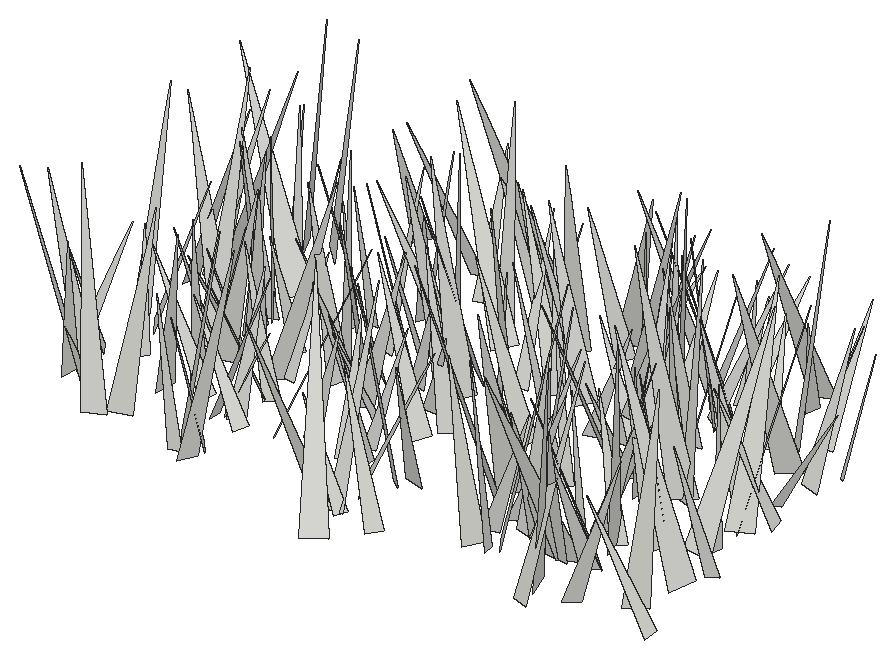
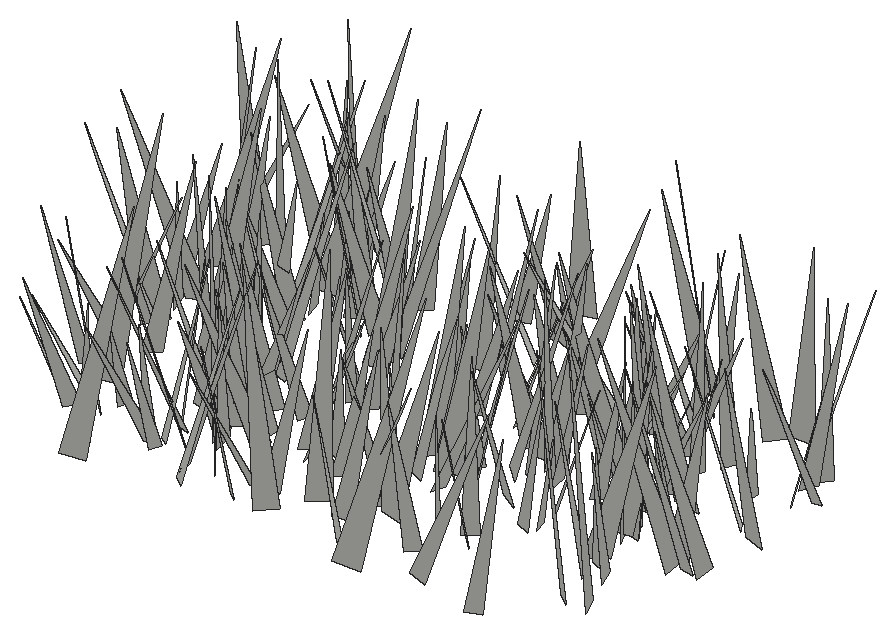
# SketchUp Ruby script. Lengths in inches.
U = 1.inch
M = Sketchup.active_model
def pt(a) = Geom::Point3d.new(a.map { |v| v * U })
def face(e, loops, mat)
  f = e.add_face(loops[0].map { |a| pt(a) })
  loops[1..].each { |l| e.add_face(l.map { |a| pt(a) }).erase! }
  f.material = f.back_material = mat if mat
  f
end
# faces: each face lists its corners as indices into pts; further lists are holes
def faces(e, pts, list, mat = nil) = list.each { |f| face(e, (f[0].is_a?(Array) ? f : [f]).map { |l| l.map { |i| pts[i] } }, mat) }
# xy, xz, yz: faces in a plane at the given z, y or x. An outline is a flat list of corners, or four numbers for a rectangle; further outlines are holes
def ring(l) = l.size == 4 ? [[l[0], l[1]], [l[2], l[1]], [l[2], l[3]], [l[0], l[3]]] : l.each_slice(2).to_a
def flat(e, list, mat, &to3) = list.each { |f| face(e, (f[0].is_a?(Array) ? f : [f]).map { |l| ring(l).map { |u, v| to3.(u, v) } }, mat) }
def xy(e, z, list, mat = nil) = flat(e, list, mat) { |x, y| [x, y, z] }
def xz(e, y, list, mat = nil) = flat(e, list, mat) { |x, z| [x, y, z] }
def yz(e, x, list, mat = nil) = flat(e, list, mat) { |y, z| [x, y, z] }
def lines(e, pts, list) = list.each { |a, b| e.add_line(pt(pts[a]), pt(pts[b])) }
# prism: a flat outline (further loops are holes) pulled along v
def prism(e, loops, v, mat = nil)
  f = face(e, loops, mat); d = Geom::Vector3d.new(v.map { |x| x * U })
  f.pushpull(f.normal.samedirection?(d) ? d.length : -d.length)
end
def box(e, o, s, mat = nil) = prism(e, [[o, [o[0] + s[0], o[1], o[2]], [o[0] + s[0], o[1] + s[1], o[2]], [o[0], o[1] + s[1], o[2]]]], [0, 0, s[2]], mat)
def at(x, y, z, deg = 0) = Geom::Transformation.translation(pt([x, y, z])) * Geom::Transformation.rotation(ORIGIN, Z_AXIS, deg.degrees)
def axes(o, x, y, z) = Geom::Transformation.new([*x, 0, *y, 0, *z, 0, *pt(o).to_a, 1])
def part(name) = M.definitions.add(name)
# library, detail: a bought-in or finely detailed component or shape, given as its bounding box
def library(name, o, s) = part(name).tap { |d| box(d.entities, o, s) }
def detail(e, o, s) = box(e.add_group.entities, o, s)
def put(e, d, t, mat = nil) = e.add_instance(d, t).tap { |i| i.material = mat if mat }
def group(e, t, mat = nil) = e.add_group.tap { |g| g.transformation = t; g.material = mat if mat }.entities
root = M.entities
c1 = part("fur_instance\#9")
p = [[0.8125,0,1.79],[0.67,-0.02,1.48],[0,-0.11,0],[0,0.11,0]]
faces(c1.entities,p,[[0,1,2,3]])
put(root,c1,axes([478.85,278.48,-21.66],[-3.36629,7.35026,0.38103],[7.33966,3.3212,0.77612],[-0.54849,-0.66835,8.0471]))
put(root,c1,axes([500.75,281.7,-21.66],[-4.62797,0.36048,0.06702],[0.36662,4.56134,0.78248],[0.00509,-0.78533,4.57556]))
put(root,c1,axes([492.17,282.21,-21.66],[7.07527,1.73735,2.55738],[2.12787,-7.36989,-0.88027],[-2.24293,-1.5114,7.23207]))
put(root,c1,axes([481.05,281.24,-21.66],[-3.33055,3.67395,0.98734],[3.8043,3.21801,0.85849],[0.0046,-1.30837,4.884]))
put(root,c1,axes([467.34,282.92,-21.66],[3.26712,2.26093,2.86418],[3.20778,-3.61207,-0.80776],[-1.73938,-2.41465,3.89016]))
put(root,c1,axes([478.22,281.67,-21.66],[-2.47066,2.78913,0.64805],[2.82871,2.24449,1.12431],[-0.44456,-1.21919,3.55237]))
put(root,c1,axes([466.3,281.52,-21.66],[-0.19493,4.51759,1.73565],[4.75586,-0.14282,0.90585],[-0.89608,-1.74071,4.43013]))
put(root,c1,axes([494.83,281.91,-21.66],[4.67154,-2.82363,0.84685],[-2.94301,-4.55853,1.0353],[-0.16964,1.32674,5.35951]))
put(root,c1,axes([467.43,281.26,-21.66],[6.54484,-1.1484,2.12677],[-1.53141,-6.71985,1.08414],[-1.86996,1.48383,6.55579]))
put(root,c1,axes([491.85,285.52,-21.66],[1.8393,-7.94223,0.20343],[-7.82957,-1.84746,-1.33722],[-1.34842,-0.10629,8.04201]))
put(root,c1,axes([465.96,282.625,-21.66],[6.04593,4.4435,2.18806],[4.86244,-5.98205,-1.28733],[-0.94282,-2.35709,7.39194]))
put(root,c1,axes([474.54,283.67,-21.66],[-1.00098,-5.50903,0.83943],[-5.47181,0.81017,-1.20786],[-1.05515,1.02481,5.46739]))
put(root,c1,axes([492.6,280.02,-21.66],[3.19327,6.60837,0.52108],[6.51338,-3.23542,1.11669],[-1.23207,0.02336,7.254]))
put(root,c1,axes([460.02,282.04,-21.66],[-1.69454,7.12423,1.83382],[7.32335,1.45532,1.11334],[-0.69716,-2.02889,7.23786]))
put(root,c1,axes([491.04,285.28,-21.66],[0.94954,-6.1364,0.24208],[-6.03443,-0.88683,1.18943],[1.14,0.41683,6.09444]))
put(root,c1,axes([486.33,283.63,-21.66],[-4.53938,3.59005,2.40826],[4.08452,4.7056,0.68422],[1.41595,-2.06469,5.74685]))
put(root,c1,axes([461.17,282.91,-21.66],[-3.27295,5.40819,2.7555],[5.57889,3.91368,-1.05481],[2.39109,-1.7286,6.23283]))
put(root,c1,axes([456.03,284.88,-21.66],[5.00192,-1.81934,1.03799],[-1.65,-5.07776,-0.94895],[-1.29032,-0.55947,5.23724]))
put(root,c1,axes([493.34,285.47,-21.66],[2.17041,-4.52553,0.56409],[-4.42394,-2.24099,-0.95709],[-1.10786,0.0828,4.92697]))
put(root,c1,axes([498.17,283.59,-21.66],[4.86014,-4.74094,2.82615],[-5.30574,-5.05065,0.65171],[-1.52079,2.46963,6.75816]))
put(root,c1,axes([457.46,284.31,-21.66],[-5.88104,-3.53705,0.94417],[-3.64814,5.81133,-0.9531],[0.30541,1.30636,6.79625]))
put(root,c1,axes([493.27,286.38,-21.66],[-4.06699,-5.2197,0.56162],[-5.13541,4.10303,0.94539],[1.09007,-0.14467,6.54919]))
put(root,c1,axes([487.39,283.66,-21.66],[-5.21816,-1.76906,1.50642],[-2.07355,5.2165,-1.05669],[1.04846,1.51216,5.4076]))
put(root,c1,axes([477.78,281.6875,-21.66],[1.53889,6.65129,0.3221],[6.53467,-1.57198,1.24039],[-1.28121,-0.02868,6.71336]))
put(root,c1,axes([488.67,286.82,-21.66],[4.29462,-4.11505,0.26594],[-3.98176,-4.23808,-1.27765],[-1.07236,-0.74374,5.80905]))
put(root,c1,axes([477.53,284.37,-21.66],[5.0651,3.0377,0.15182],[3.00547,-4.95362,-1.15532],[0.46672,-1.0677,5.79207]))
put(root,c1,axes([490.27,285.51,-21.66],[-1.57238,-4.56901,1.11948],[-4.65933,1.35009,-1.0341],[-0.64787,1.37945,4.72005]))
put(root,c1,axes([479.28,287,-21.66],[-0.0268,-5.65268,0.22398],[-5.53849,0.07185,1.15049],[1.15241,0.21383,5.53443]))
put(root,c1,axes([486.15,285.42,-21.66],[3.07396,-3.53335,0.83024],[-3.61315,-2.87553,1.13994],[0.34489,1.36741,4.5425]))
put(root,c1,axes([456.26,286.05,-21.66],[-6.02827,1.48886,1.73676],[1.72693,6.17226,0.7029],[1.50026,-1.12234,6.1695]))
put(root,c1,axes([461.34,286.85,-21.66],[5.97247,-1.71505,1.0533],[-1.60325,-6.04797,-0.7569],[-1.21673,-0.44932,6.16757]))
put(root,c1,axes([467.66,285.83,-21.66],[-3.1989,2.68909,0.37978],[2.66785,3.00183,1.21655],[-0.50792,-1.16886,3.99802]))
put(root,c1,axes([487.98,286.3,-21.66],[-0.07815,-6.05054,2.52953],[-6.4447,0.53908,1.09033],[1.2138,2.47266,5.952]))
put(root,c1,axes([487.625,284.45,-21.66],[6.38887,5.18246,1.59043],[5.07791,-6.58181,1.04866],[-1.89794,-0.16426,8.1594]))
put(root,c1,axes([497.56,287.66,-21.66],[4.54557,4.08977,3.87164],[5.12111,-5.0718,-0.65499],[-2.34307,-3.15097,6.07942]))
put(root,c1,axes([478.53,286.3125,-21.66],[2.96491,4.33641,3.25393],[4.46173,-4.05854,1.34327],[-3.07985,-1.70497,5.07846]))
put(root,c1,axes([484.5,288.24,-21.66],[-4.58981,-6.81856,1.14154],[-6.9132,4.53833,-0.68805],[0.05895,1.33156,8.19058]))
put(root,c1,axes([465.78,286.79,-21.66],[3.19259,1.80159,0.09548],[1.75198,-3.04965,-1.03811],[0.43061,-0.9494,3.51578]))
put(root,c1,axes([498.67,287.17,-21.66],[-7.81883,2.51294,1.68172],[2.76611,7.82758,1.16397],[1.22135,-1.64052,8.12983]))
put(root,c1,axes([471.63,287.34,-21.66],[1.56073,-4.1385,0.9971],[-4.17951,-1.28812,1.1957],[0.80812,1.33073,4.25833]))
put(root,c1,axes([465.54,286.11,-21.66],[4.89085,0.64493,0.58721],[0.56841,-4.89366,0.64042],[-0.66156,0.56328,4.89144]))
put(root,c1,axes([466.84,286.4375,-21.66],[-2.42701,4.03219,1.90827],[4.11447,2.86278,-0.81615],[1.72373,-1.15601,4.63496]))
put(root,c1,axes([484.32,289.6,-21.66],[5.05065,-5.78899,0.88016],[-5.66798,-5.12516,-1.18448],[-1.47008,-0.1285,7.59069]))
put(root,c1,axes([486.57,287.27,-21.66],[4.08139,-3.20586,0.61223],[-3.2526,-3.91407,1.18774],[0.27008,1.30866,5.05219]))
put(root,c1,axes([455.82,288.23,-21.66],[-3.08221,-2.2445,0.63722],[-2.14243,3.14072,0.69983],[0.92405,-0.20483,3.74807]))
put(root,c1,axes([463.95,287.48,-21.66],[-4.51711,1.79985,0.33219],[1.82954,4.41557,0.95372],[-0.05124,-1.00862,4.76803]))
put(root,c1,axes([464.62,285.65,-21.66],[4.77639,3.07128,1.21309],[2.81816,-4.90311,1.31748],[-1.72115,0.49496,5.52367]))
put(root,c1,axes([492.72,288.47,-21.66],[7.08469,1.17747,2.52447],[1.61288,-7.35894,-1.094],[-2.27113,-1.55299,7.09806]))
put(root,c1,axes([475.82,287.45,-21.66],[-4.15206,-1.52587,0.16301],[-1.50616,3.96212,-1.27574],[-0.29385,1.25209,4.2356]))
put(root,c1,axes([462.26,288.76,-21.66],[5.48977,-0.87036,1.92832],[-0.64898,-5.79667,-0.76876],[-2.01365,-0.50463,5.50492]))
put(root,c1,axes([454.75,287.21,-21.66],[1.35315,4.35582,0.79538],[4.34518,-1.14634,-1.11449],[0.85157,-1.07217,4.42291]))
put(root,c1,axes([474.34,286.75,-21.66],[-3.56654,2.39752,0.7344],[2.22273,3.6139,-1.00345],[1.16058,0.44646,4.17868]))
put(root,c1,axes([499.32,289.1,-21.66],[0.38107,-4.3176,1.24457],[-4.35966,-0.65774,-0.94692],[-1.08815,1.12319,4.22969]))
put(root,c1,axes([491.2,287.46,-21.66],[-4.4304,-0.23548,0.66281],[-0.42328,4.26855,-1.31284],[0.56178,1.35914,4.23796]))
put(root,c1,axes([469.55,286.65,-21.66],[5.6659,3.07924,0.02777],[3.03508,-5.59401,1.03936],[-0.52039,0.90013,6.36426]))
put(root,c1,axes([491.08,289.32,-21.66],[4.31446,-3.71791,0.40504],[-3.72385,-4.21342,0.9907],[0.3462,1.01276,5.60856]))
put(root,c1,axes([487.67,287.64,-21.66],[-4.49953,-3.59508,3.80394],[-4.60675,5.10137,-0.62788],[2.48443,2.94818,5.72505]))
put(root,c1,axes([494.8125,289.5625,-21.66],[4.62611,-3.05223,2.53258],[-2.97331,-5.24406,-0.88892],[-2.62479,0.5609,5.47054]))
put(root,c1,axes([492.79,288.73,-21.66],[1.4221,-3.78822,2.5832],[-4.25079,-2.10312,-0.74405],[-1.71882,2.06693,3.97736]))
put(root,c1,axes([466.5,289.45,-21.66],[-2.71564,-2.49022,0.0198],[-2.39499,2.6036,-1.03032],[-0.68234,0.77224,3.53756]))
put(root,c1,axes([473.71,290.93,-21.66],[-3.49973,-1.74713,0.54329],[-1.50598,3.41664,1.28623],[1.03907,-0.93268,3.69408]))
put(root,c1,axes([474.87,288.43,-21.66],[3.51726,-1.23078,1.44078],[-1.67757,-3.4351,1.16087],[-0.88116,1.62697,3.54095]))
put(root,c1,axes([467.04,289.42,-21.66],[1.69917,-3.99461,2.49122],[-4.30676,-2.38859,-0.89256],[-1.90128,1.84064,4.24822]))
put(root,c1,axes([484.5,290.53,-21.66],[0.91416,-4.94391,1.27953],[-4.9749,-1.15567,-0.91103],[-1.1532,1.06645,4.94449]))
put(root,c1,axes([458.07,288.97,-21.66],[-3.61922,1.27993,0.57976],[1.16278,3.62754,-0.74965],[0.78884,0.52519,3.76496]))
put(root,c1,axes([461.9,291.4,-21.66],[4.17452,-5.37379,1.20818],[-5.50555,-4.02647,1.11376],[0.16212,1.6352,6.71296]))
put(root,c1,axes([489.99,291.05,-21.66],[3.34433,-2.45993,0.06359],[-2.39384,-3.22746,1.0454],[0.56992,0.87868,4.01783]))
put(root,c1,axes([460.62,292.15,-21.66],[-3.9819,-2.09854,0.99873],[-1.89028,4.07705,1.03024],[1.35209,-0.4803,4.38155]))
put(root,c1,axes([470.4375,292.9,-21.66],[1.77342,-4.13167,0.71101],[-4.001,-1.89854,-1.053],[-1.2523,0.21471,4.37115]))
put(root,c1,axes([476.4,291.35,-21.66],[-4.85696,2.92878,0.85344],[3.03677,4.79447,0.82904],[0.29007,-1.15391,5.61075]))
put(root,c1,axes([462.3,292.6875,-21.66],[-0.70477,-3.63934,0.22038],[-3.52996,0.62491,-0.96896],[-0.91253,0.39339,3.57807]))
put(root,c1,axes([463.36,291.9375,-21.66],[-3.08913,-1.9262,0.20442],[-1.91689,2.98464,-0.84391],[-0.27849,0.82245,3.5413]))
put(root,c1,axes([465.73,291.59,-21.66],[6.31096,-2.97385,1.65761],[-3.28181,-6.24286,1.29466],[-0.9062,1.89806,6.85536]))
put(root,c1,axes([487.78,294.82,-21.66],[-3.38776,-6.42257,0.32475],[-6.36234,3.40084,0.88702],[0.93573,-0.12917,7.20691]))
put(root,c1,axes([456.41,292.04,-21.66],[4.70564,3.18962,0.73071],[3.27223,-4.59158,-1.02983],[-0.01227,-1.26267,5.59072]))
put(root,c1,axes([471.5,292.12,-21.66],[4.65487,-3.05281,1.35089],[-3.29302,-4.57961,0.99778],[-0.54826,1.58741,5.47649]))
put(root,c1,axes([466.07,291.91,-21.66],[-0.49271,4.25835,1.65602],[4.30491,0.99075,-1.26683],[1.53091,-1.41548,4.0953]))
put(root,c1,axes([490.07,294.01,-21.66],[3.94789,-1.4658,0.35037],[-1.34081,-3.86465,-1.06014],[-0.68816,-0.87925,4.0756]))
put(root,c1,axes([468.7,293.47,-21.66],[-5.74569,2.33772,2.68731],[2.89131,6.03979,0.92776],[2.08013,-1.9379,6.13328]))
put(root,c1,axes([497.58,291.7,-21.66],[-4.70779,-0.34884,1.44292],[-0.70643,4.74641,-1.15738],[1.30563,1.3103,4.57662]))
put(root,c1,axes([462.11,294.08,-21.66],[1.6892,-5.96403,1.00433],[-6.01842,-1.55459,0.89085],[0.59746,1.20222,6.13428]))
put(root,c1,axes([496.96,290.64,-21.66],[-0.59068,7.87895,1.19707],[7.83923,0.79048,-1.33468],[1.43434,-1.07565,7.78752]))
put(root,c1,axes([483.6,292.64,-21.66],[2.51167,3.62255,0.80621],[3.69421,-2.34748,-0.96099],[0.35452,-1.20325,4.30208]))
put(root,c1,axes([477.14,292.81,-21.66],[1.60632,-4.77246,2.92285],[-5.28453,-2.29441,-0.84211],[-1.84207,2.42054,4.96463]))
put(root,c1,axes([469.46,294.94,-21.66],[-2.94569,-5.43055,1.36405],[-5.282,3.20651,1.35919],[1.85796,0.50597,6.02666]))
put(root,c1,axes([474.76,294.08,-21.66],[1.46313,-3.34357,0.17988],[-3.25058,-1.37123,0.95187],[0.80348,0.54115,3.52337]))
put(root,c1,axes([488.31,293.77,-21.66],[4.57096,2.53062,0.74602],[2.63797,-4.36083,-1.37058],[0.04077,-1.55993,5.04174]))
put(root,c1,axes([482.78,294.48,-21.66],[3.65052,-1.24636,0.3015],[-1.17659,-3.61738,-0.70767],[-0.50984,-0.576,3.79195]))
put(root,c1,axes([486.3125,292.16,-21.66],[-4.58917,0.765,0.19448],[0.68534,4.43094,-1.25723],[0.3916,1.21042,4.47941]))
put(root,c1,axes([464.78,294.58,-21.66],[3.15907,-2.58161,1.45094],[-2.40771,-3.47422,-0.93937],[-1.72421,0.12146,3.97014]))
put(root,c1,axes([461.76,294.01,-21.66],[2.13967,5.72529,2.72362],[6.33838,-1.99885,-0.77766],[-0.14822,-2.82858,6.06237]))
put(root,c1,axes([484.8,293.13,-21.66],[-6.17227,-0.98801,0.5453],[-1.07692,6.06305,-1.2042],[0.3373,1.27815,6.13375]))
put(root,c1,axes([488.39,295.1,-21.66],[0.67909,-3.62862,0.46379],[-3.53581,-0.77205,-0.86319],[-0.93808,0.2832,3.58928]))
put(root,c1,axes([481.48,294.62,-21.66],[-5.50696,2.25656,1.40845],[2.52369,5.45565,1.12666],[0.84072,-1.59571,5.84374]))
put(root,c1,axes([492.36,295.125,-21.66],[2.49125,-7.31611,3.2771],[-7.62751,-3.2193,-1.38865],[-2.46697,2.5655,7.60286]))
put(root,c1,axes([470.43,295.32,-21.66],[-4.6315,-5.30606,1.24554],[-5.44783,4.55599,-0.84886],[0.16366,1.49838,6.99175]))
put(root,c1,axes([460.3,292.1,-21.66],[0.64716,8.27924,1.09317],[8.31403,-0.74193,0.69715],[-0.78591,-1.0312,8.27518]))
put(root,c1,axes([461.21,295.34,-21.66],[2.3019,2.88607,2.09295],[3.52279,-2.224,-0.8077],[-0.54756,-2.17555,3.60219]))
put(root,c1,axes([454.7,293.02,-21.66],[1.29784,6.7007,1.25957],[6.74597,-1.44798,0.75208],[-0.98888,-1.08363,6.78367]))
put(root,c1,axes([468.62,294.11,-21.66],[2.86323,5.98862,2.41998],[6.20716,-3.28322,0.78076],[-1.78634,-1.80966,6.59182]))
put(root,c1,axes([498.45,295.98,-21.66],[-4.68733,-0.90911,0.30449],[-0.85582,4.65242,0.7161],[0.43216,-0.64711,4.72067]))
put(root,c1,axes([472.43,295.88,-21.66],[0.98375,-3.96673,0.69714],[-3.91068,-0.76919,1.14174],[0.96305,0.9285,3.92417]))
put(root,c1,axes([467.69,294.625,-21.66],[-5.58164,-0.15602,0.84627],[-0.25003,5.60842,-0.61509],[0.82341,0.64537,5.54984]))
put(root,c1,axes([460.52,296.74,-21.66],[-2.8459,-6.01928,1.64103],[-5.98512,3.14324,1.14988],[1.76154,0.95508,6.5581]))
put(root,c1,axes([472.79,295.42,-21.66],[-4.95008,-4.07189,1.35786],[-4.2827,4.82407,-1.14641],[0.2873,1.75371,6.30629]))
put(root,c1,axes([474.5,296.41,-21.66],[-2.85824,2.70123,1.97363],[3.21945,2.92659,0.65696],[0.90938,-1.87078,3.87745]))
put(root,c1,axes([487.84,296.85,-21.66],[3.54062,0.10617,1.20258],[0.38468,-3.63127,-0.812],[-1.14433,-0.89222,3.44788]))
put(root,c1,axes([465.68,297.39,-21.66],[-3.61169,-1.5954,0.61372],[-1.41522,3.59542,1.01805],[0.9587,-0.70282,3.81487]))
put(root,c1,axes([497.0625,294.25,-21.66],[6.03648,4.13261,1.07509],[4.02235,-6.12795,0.97074],[-1.43354,0.20766,7.25088]))
put(root,c1,axes([495.21,297.11,-21.66],[4.87258,-2.82126,2.84071],[-2.53321,-5.63755,-1.25383],[-3.10033,0.17232,5.48903]))
put(root,c1,axes([475.28,296.43,-21.66],[-6.5147,3.53544,2.59254],[3.94464,6.75335,0.70282],[1.91322,-1.88542,7.3788]))
put(root,c1,axes([492.85,294.8,-21.66],[2.9733,6.47594,2.08154],[6.51847,-3.36189,1.14821],[-1.94427,-1.36785,7.03277]))
put(root,c1,axes([460.88,296.75,-21.66],[1.22573,-5.85041,2.29876],[-6.17569,-1.55733,-0.67049],[-1.1715,2.08841,5.93971]))
put(root,c1,axes([473.35,297.53,-21.66],[3.66547,-5.8791,2.24711],[-5.89364,-4.11869,-1.16204],[-2.20868,1.23351,6.83002]))
put(root,c1,axes([460.84,297.32,-21.66],[5.57047,2.74276,2.66238],[3.42235,-5.67452,-1.31471],[-1.7025,-2.43273,6.06831]))
put(root,c1,axes([497.28,294.17,-21.66],[-5.06165,5.7028,1.49455],[5.55918,5.27278,-1.292],[1.96243,-0.22764,7.51486]))
put(root,c1,axes([474.52,298.93,-21.66],[-3.9391,-6.11846,0.96009],[-6.01065,4.05101,1.1555],[1.49311,0.1661,7.18449]))
put(root,c1,axes([457.06,296.97,-21.66],[1.7878,3.1828,1.34143],[3.44443,-1.53093,-0.95817],[0.2561,-1.62848,3.52255]))
put(root,c1,axes([489.68,297.91,-21.66],[-1.49561,-5.63035,1.67127],[-5.71638,1.79132,0.91926],[1.34798,1.34949,5.75262]))
put(root,c1,axes([470.625,298.5625,-21.66],[-3.85431,-2.63258,1.04926],[-2.43046,3.98156,1.06172],[1.4575,-0.32233,4.54521]))
put(root,c1,axes([485.56,297.93,-21.66],[2.4486,-4.30122,0.69777],[-4.269,-2.2075,1.37318],[0.8735,1.26866,4.75506]))
put(root,c1,axes([457.02,297.09,-21.66],[-2.59565,5.50063,1.7013],[5.74289,2.3395,1.19781],[-0.41302,-2.03926,5.96319]))
put(root,c1,axes([487.13,297.68,-21.66],[-3.1283,2.85302,0.75954],[2.94685,2.94951,1.058],[-0.18092,-1.28978,4.09959]))
put(root,c1,axes([483.6875,297.57,-21.66],[3.11489,-2.67244,0.85057],[-2.80172,-2.90834,1.1224],[0.12545,1.40269,3.94774]))
put(root,c1,axes([488.51,296.26,-21.66],[-5.11212,3.73872,1.49873],[3.53116,5.32488,-1.23875],[1.93782,0.15985,6.21106]))
put(root,c1,axes([454.67,297.48,-21.66],[6.22243,-0.20354,0.93497],[-0.30289,-6.25415,0.65425],[-0.90767,0.69164,6.19128]))
put(root,c1,axes([476.15,299.46,-21.66],[-2.86307,-5.78602,1.82095],[-5.78172,3.21211,1.11581],[1.83453,1.09334,6.35847]))
put(root,c1,axes([472.6,299.3,-21.66],[-6.27523,-0.24227,0.55286],[-0.1392,6.19931,1.13667],[0.58735,-1.11924,6.17618]))
put(root,c1,axes([497.02,297.79,-21.66],[3.6219,-1.04912,0.12415],[-1.02885,-3.40219,1.26523],[0.23987,1.24847,3.55218]))
put(root,c1,axes([495.21,301.28,-21.66],[3.52334,-7.25518,1.10129],[-7.15699,-3.66725,-1.26216],[-1.62106,0.42196,7.96608]))
put(root,c1,axes([476.77,297.96,-21.66],[1.67627,3.15128,1.04901],[3.10636,-1.90337,0.75402],[-1.17538,-0.53615,3.48882]))
put(root,c1,axes([455.6,297.99,-21.66],[2.77668,6.00015,1.42785],[6.14966,-2.57364,-1.14395],[0.47149,-1.76779,6.51177]))
put(root,c1,axes([456.45,298,-21.66],[7.58645,0.4489,1.20084],[0.2907,-7.62155,1.01257],[-1.24861,0.95304,7.53196]))
put(root,c1,axes([465.38,299.07,-21.66],[-3.65849,-0.26653,0.63033],[-0.40108,3.61269,-0.80033],[0.55452,0.85461,3.57982]))
put(root,c1,axes([468.625,297.9,-21.66],[1.97963,5.14738,0.61551],[5.06452,-2.06097,0.94673],[-1.10678,-0.22402,5.43306]))
put(root,c1,axes([466.03,299.85,-21.66],[-1.43157,-3.77915,1.63266],[-4.11341,1.2436,-0.72817],[-0.16553,1.78,3.97506]))
put(root,c1,axes([489.01,300.27,-21.66],[-0.52973,-5.32119,2.08202],[-5.65742,0.19488,-0.94137],[-0.8022,2.1395,5.26399]))
put(root,c1,axes([489.66,298.7,-21.66],[4.69636,2.95892,0.9191],[2.85112,-4.78039,0.82137],[-1.21287,0.21986,5.48965]))
put(root,c1,axes([481.15,300.29,-21.66],[-4.7653,3.97573,1.88545],[4.327,4.73874,0.94381],[0.79899,-1.95123,6.13381]))
put(root,c1,axes([460.6,299.96,-21.66],[-6.11884,4.72961,1.11538],[4.85918,5.97068,1.339],[0.0418,-1.7422,7.61686]))
put(root,c1,axes([467.91,302.25,-21.66],[4.2644,-2.86076,0.08373],[-2.8192,-4.22473,-0.76148],[-0.49304,-0.58632,5.07831]))
put(root,c1,axes([486.15,300.71,-21.66],[-1.6675,3.7386,1.84502],[3.94069,2.06209,-0.61692],[1.36097,-1.39013,4.04687]))
put(root,c1,axes([480.8125,300.8,-21.66],[-5.83458,-0.97839,0.23219],[-1.00024,5.78729,-0.74851],[0.10327,0.77686,5.8685]))
put(root,c1,axes([459.8,301.95,-21.66],[5.00049,1.26706,0.71261],[1.41038,-4.84715,-1.27832],[-0.35226,-1.4205,4.99762]))
put(root,c1,axes([483.9,300.7,-21.66],[7.6269,-0.50277,1.8471],[-0.68475,-7.80192,0.70374],[-1.78765,0.84341,7.61099]))
put(root,c1,axes([497.23,300.5,-21.66],[0.7475,5.23214,1.319],[5.34274,-0.53135,-0.92008],[0.75507,-1.41992,5.20456]))
put(root,c1,axes([486.23,299.77,-21.66],[-5.56085,2.56326,1.5764],[2.25423,5.74256,-1.38556],[1.99343,0.65656,5.96435]))
put(root,c1,axes([479.32,300.09,-21.66],[-0.14147,5.00237,0.6936],[4.87308,-0.04695,1.33257],[-1.32587,-0.70632,4.82369]))
put(root,c1,axes([477.17,299.35,-21.66],[0.66443,5.27954,0.01832],[5.19176,-0.65673,0.9642],[-0.95891,0.10252,5.2331]))
put(root,c1,axes([486.18,302.52,-21.66],[7.03768,2.72348,2.80411],[3.28727,-7.24831,-1.21043],[-2.11523,-2.20318,7.44856]))
put(root,c1,axes([477.89,301.53,-21.66],[-4.17135,3.80631,1.04328],[3.93898,4.10999,0.75433],[0.24669,-1.26356,5.59635]))
put(root,c1,axes([459.77,300.73,-21.66],[0.78619,5.10987,0.99795],[4.99569,-1.02461,1.31074],[-1.46621,-0.75112,5.00108]))
put(root,c1,axes([484.43,301.3125,-21.66],[-4.83197,-1.5354,1.95575],[-2.0901,4.8234,-1.3772],[1.34681,1.9768,4.87942]))
put(root,c1,axes([458.76,301.4,-21.66],[-4.7564,-0.43454,1.78324],[-0.95829,4.81251,-1.3833],[1.56539,1.62573,4.5715]))
put(root,c1,axes([488.3,304.64,-21.66],[-3.60567,-4.25836,0.82426],[-4.10665,3.69659,1.13335],[1.39586,-0.12438,5.46351]))
put(root,c1,axes([488.5625,302.73,-21.66],[3.89411,3.28531,3.07479],[3.51498,-4.75969,0.63397],[-2.80935,-1.40135,5.05524]))
put(root,c1,axes([477.09,304.58,-21.66],[5.45655,-4.97036,1.37233],[-4.9464,-5.60993,-0.6508],[-1.45634,0.43117,7.35221]))
put(root,c1,axes([483.26,301.95,-21.66],[6.3266,0.04535,0.7535],[-0.10627,-6.24313,1.26797],[-0.74735,1.27161,6.1984]))
put(root,c1,axes([473.5,302.51,-21.66],[-6.02819,4.2729,0.70004],[4.32885,5.97346,0.81585],[0.09372,-1.07093,7.34378]))
put(root,c1,axes([486.41,301.68,-21.66],[-2.91269,3.59929,0.76549],[3.33369,2.99435,-1.39463],[1.55801,0.3218,4.41516]))
put(root,c1,axes([485.46,302.79,-21.66],[-5.53054,0.45224,1.5037],[0.10523,5.59989,-1.29715],[1.5667,1.22031,5.39525]))
put(root,c1,axes([498.01,302.51,-21.66],[2.52886,2.74781,0.4271],[2.47453,-2.48701,1.34889],[-1.2687,0.62635,3.48225]))
put(root,c1,axes([488.21,302.99,-21.66],[2.55836,5.15566,0.46861],[5.11042,-2.43162,-1.14739],[0.82709,-0.92305,5.63999]))
put(root,c1,axes([492.64,302.73,-21.66],[-3.06168,2.49465,0.02952],[2.42804,2.99025,-0.87237],[0.57338,0.65813,3.85176]))
put(root,c1,axes([474.75,305.39,-21.66],[1.57492,-4.967,1.49516],[-5.0252,-1.8484,-0.84719],[-1.28605,1.13987,5.14138]))
put(root,c1,axes([457.36,304.64,-21.66],[6.90611,3.10223,2.59996],[3.46907,-7.18559,-0.64093],[-2.08547,-1.6797,7.5437]))
put(root,c1,axes([467.46,303.14,-21.66],[2.96652,3.66752,1.13191],[3.55325,-3.16507,0.94281],[-1.45132,-0.25254,4.62191]))
put(root,c1,axes([459.15,304.81,-21.66],[-4.14785,-5.45032,3.6874],[-5.74845,5.12259,1.10541],[3.20285,2.13555,6.75935]))
put(root,c1,axes([472.67,303.52,-21.66],[0.75585,6.87514,1.87347],[7.05211,-0.99202,0.79528],[-1.02238,-1.75986,6.87069]))
put(root,c1,axes([479.79,305.66,-21.66],[3.58153,-3.37168,2.12142],[-3.21603,-4.13077,-1.13573],[-2.3507,0.51427,4.78599]))
put(root,c1,axes([485.39,306.39,-21.66],[-6.52757,-2.25287,1.08541],[-2.07972,6.57544,1.14066],[1.38863,-0.74224,6.81054]))
put(root,c1,axes([468.82,304.05,-21.66],[3.80015,2.05854,2.10545],[1.83657,-4.34391,0.93228],[-2.30164,-0.0674,4.22014]))
put(root,c1,axes([495.16,303.01,-21.66],[3.38702,2.66566,0.2184],[2.51461,-3.29384,1.20529],[-0.91115,0.81867,4.13823]))
put(root,c1,axes([486.77,304.54,-21.66],[4.58071,3.98416,0.78034],[4.05613,-4.44078,-1.1369],[0.17387,-1.36793,5.96354]))
put(root,c1,axes([489.7,304.17,-21.66],[-4.04138,0.55951,1.25439],[0.25517,4.13619,-1.02282],[1.34961,0.89343,3.94964]))
put(root,c1,axes([493.64,303.89,-21.66],[4.42049,5.15695,1.86392],[5.12768,-4.73588,0.94203],[-1.94301,-0.76574,6.72662]))
put(root,c1,axes([478.75,307.25,-21.66],[3.49272,-6.19271,0.17705],[-6.11252,-3.41157,1.25629],[1.00898,0.76914,6.99789]))
put(root,c1,axes([484.67,307.82,-21.66],[-4.07639,-4.57708,0.71562],[-4.52519,4.13816,0.69067],[0.99219,0.06853,6.09012]))
put(root,c1,axes([494.95,304.68,-21.66],[-1.9043,4.31856,1.08738],[4.14528,2.15112,-1.28374],[1.62757,-0.42591,4.54184]))
put(root,c1,axes([488.14,305.61,-21.66],[-2.24113,2.46388,1.48853],[2.36542,2.65133,-0.82724],[1.6405,-0.45695,3.22631]))
put(root,c1,axes([491.23,309.32,-21.66],[2.31085,-7.14722,0.11909],[-7.10013,-2.30949,-0.83147],[-0.82765,-0.14321,7.46535]))
put(root,c1,axes([483.9375,305.49,-21.66],[2.37526,2.53476,1.46683],[2.25858,-2.78775,1.16004],[-1.86424,-0.14786,3.27432]))
put(root,c1,axes([481.07,305.5,-21.66],[1.22352,3.80068,0.33063],[3.61313,-1.04295,-1.38167],[1.22465,-0.72012,3.74608]))
put(root,c1,axes([473.85,305.6875,-21.66],[-6.46685,-0.99912,0.02995],[-0.985,6.33639,-1.3035],[-0.17003,1.29271,6.41243]))
put(root,c1,axes([469.26,305.78,-21.66],[-2.32023,4.26891,1.78267],[4.38145,2.66784,-0.68595],[1.48474,-1.20167,4.81004]))
put(root,c1,axes([491.71,307.73,-21.66],[3.65469,-1.69105,0.3912],[-1.57801,-3.61693,-0.89287],[-0.72291,-0.65395,3.92673]))
put(root,c1,axes([467.07,308.13,-21.66],[-0.62326,-5.57048,0.69706],[-5.46922,0.44429,-1.33972],[-1.26641,0.82277,5.44278]))
put(root,c1,axes([473.33,307.4,-21.66],[4.06757,1.21437,0.51699],[1.31683,-3.847,-1.32426],[-0.08902,-1.4188,4.03313]))
put(root,c1,axes([471.11,309.55,-21.66],[1.71301,-8.16044,0.92704],[-8.06805,-1.84913,-1.36891],[-1.53583,0.61199,8.22516]))
put(root,c1,axes([488.8,305.16,-21.66],[-0.26739,4.57604,0.32256],[4.40279,0.34673,-1.26925],[1.2883,-0.2352,4.40462]))
put(root,c1,axes([481.2,307.29,-21.66],[3.19088,3.17646,1.19509],[3.39239,-3.03309,-0.99593],[-0.09903,-1.55252,4.39087]))
put(root,c1,axes([462.09,309.27,-21.66],[3.35364,-3.87615,0.32814],[-3.76663,-3.34394,-1.00479],[-0.97195,-0.41544,5.02611]))
